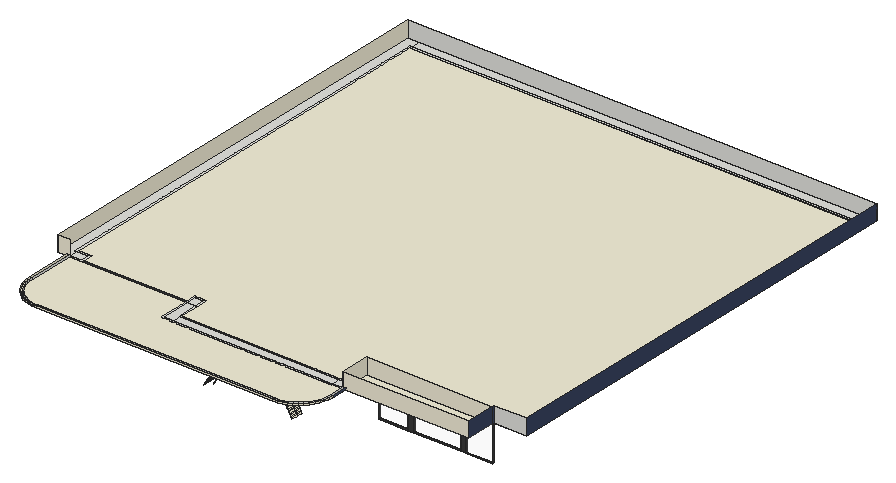
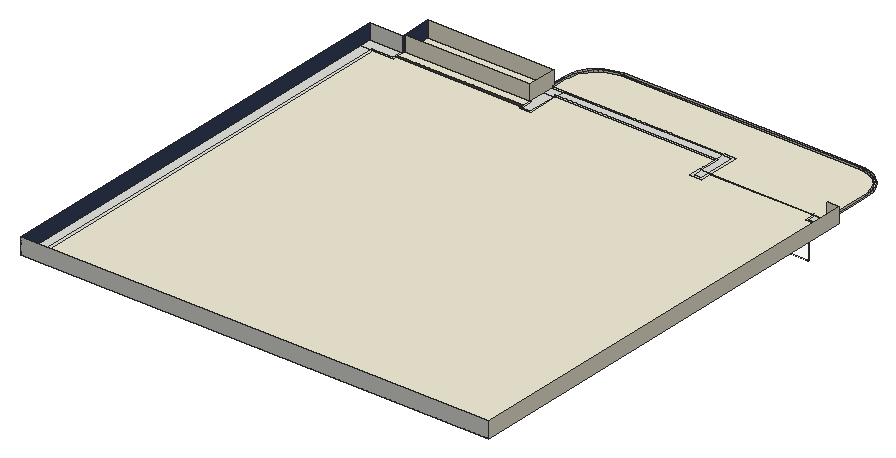
# SketchUp Ruby script. Lengths in inches.
U = 1.inch
M = Sketchup.active_model
def pt(a) = Geom::Point3d.new(a.map { |v| v * U })
def face(e, loops, mat)
  f = e.add_face(loops[0].map { |a| pt(a) })
  loops[1..].each { |l| e.add_face(l.map { |a| pt(a) }).erase! }
  f.material = f.back_material = mat if mat
  f
end
# faces: each face lists its corners as indices into pts; further lists are holes
def faces(e, pts, list, mat = nil) = list.each { |f| face(e, (f[0].is_a?(Array) ? f : [f]).map { |l| l.map { |i| pts[i] } }, mat) }
# xy, xz, yz: faces in a plane at the given z, y or x. An outline is a flat list of corners, or four numbers for a rectangle; further outlines are holes
def ring(l) = l.size == 4 ? [[l[0], l[1]], [l[2], l[1]], [l[2], l[3]], [l[0], l[3]]] : l.each_slice(2).to_a
def flat(e, list, mat, &to3) = list.each { |f| face(e, (f[0].is_a?(Array) ? f : [f]).map { |l| ring(l).map { |u, v| to3.(u, v) } }, mat) }
def xy(e, z, list, mat = nil) = flat(e, list, mat) { |x, y| [x, y, z] }
def xz(e, y, list, mat = nil) = flat(e, list, mat) { |x, z| [x, y, z] }
def yz(e, x, list, mat = nil) = flat(e, list, mat) { |y, z| [x, y, z] }
def lines(e, pts, list) = list.each { |a, b| e.add_line(pt(pts[a]), pt(pts[b])) }
# prism: a flat outline (further loops are holes) pulled along v
def prism(e, loops, v, mat = nil)
  f = face(e, loops, mat); d = Geom::Vector3d.new(v.map { |x| x * U })
  f.pushpull(f.normal.samedirection?(d) ? d.length : -d.length)
end
def box(e, o, s, mat = nil) = prism(e, [[o, [o[0] + s[0], o[1], o[2]], [o[0] + s[0], o[1] + s[1], o[2]], [o[0], o[1] + s[1], o[2]]]], [0, 0, s[2]], mat)
def at(x, y, z, deg = 0) = Geom::Transformation.translation(pt([x, y, z])) * Geom::Transformation.rotation(ORIGIN, Z_AXIS, deg.degrees)
def axes(o, x, y, z) = Geom::Transformation.new([*x, 0, *y, 0, *z, 0, *pt(o).to_a, 1])
def part(name) = M.definitions.add(name)
# library, detail: a bought-in or finely detailed component or shape, given as its bounding box
def library(name, o, s) = part(name).tap { |d| box(d.entities, o, s) }
def detail(e, o, s) = box(e.add_group.entities, o, s)
def put(e, d, t, mat = nil) = e.add_instance(d, t).tap { |i| i.material = mat if mat }
def group(e, t, mat = nil) = e.add_group.tap { |g| g.transformation = t; g.material = mat if mat }.entities
root = M.entities
M.materials.add("0344 AP 9635 Ganges Midnight-N").color = [69, 80, 105]
M.materials.add("0360 AP 9644 Monsoon Midnight-N").color = [56, 67, 95]
M.materials.add("0905 AP 7844 MILD YELLOW").color = [242, 237, 215]
M.materials.add("Glass Clear 001").color = [246, 246, 246]
M.materials["Glass Clear 001"].alpha = 0.1
M.materials.add("[Color M07]").color = [58, 58, 58]
xy(root,86.69,[[46.79,89.9375,64.29,90.25],[67.49,89.9375,95.54,90.25],[98.74,89.9375,118.39,90.25]],"[Color M07]")
xy(root,88.49,[[266.94,94.4375,289.69,95.5],[293.7,94.4375,329.88,95.5],[334.04,94.4375,354.52,95.5]],"[Color M07]")
xy(root,115.63,[[266.94,94.4375,289.69,95.5],[293.7,94.4375,329.88,95.5],[334.04,94.4375,354.52,95.5]])
xy(root,116.26,[[46.79,89.9375,64.29,90.25],[67.49,89.9375,95.54,90.25],[98.74,89.9375,118.39,90.25]])
xy(root,120,[[122.125,65.9375,131.125,65.9375,131.125,67.61,123.8,67.61,123.8,89.9375,122.125,89.9375],[131.125,65.9375,253.5625,67.61],[253.5625,65.9375,262.5625,67.61],[123.8,67.61,131.125,67.61,131.125,73.27,129.45,73.27,129.45,89.9375,123.8,89.9375],[131.125,67.61,253.5625,73.27],
  [253.5625,67.61,262.5625,67.61,262.5625,74.9375,255.23,74.9375,255.23,73.27,253.5625,73.27],[129.45,73.27,131.125,89.9375],[131.125,73.27,253.5625,74.9375],[253.5625,73.27,255.23,74.9375],[253.5625,74.9375,255.23,74.9375,255.23,97.27,260.89,97.27,260.89,88.27,262.5625,88.27,262.5625,98.9375,253.5625,98.9375],
  [255.23,74.9375,262.5625,74.9375,262.5625,88.27,260.89,88.27,260.89,97.27,255.23,97.27],[358.89,88.27,360.57,89.9375],[24,89.9375,31.33,89.9375,31.33,91.61,33,91.61,33,97.27,31.33,97.27,31.33,418.61,33,418.61,33,425.9375,24,425.9375],[31.33,89.9375,33,91.61],[33,89.9375,33,91.61,41.38,91.61,41.38,97.27,33,97.27,33,98.9375,43.05,98.9375,43.05,89.9375],
  [122.125,89.9375,122.125,98.9375,131.125,98.9375,131.125,89.9375,129.45,89.9375,129.45,97.27,123.8,97.27,123.8,89.9375],[123.8,89.9375,129.45,97.27],[358.89,89.9375,358.89,98.9375,376.67,98.9375,376.67,97.27,360.57,97.27,360.57,89.9375],[360.57,89.9375,360.57,97.27,376.67,97.27,376.67,98.9375,384,98.9375,384,89.9375],[33,91.61,41.38,97.27],
  [31.33,97.27,33,418.61],[375,98.9375,376.67,416.9375],[376.67,98.9375,384,416.9375],[33,416.9375,376.67,418.61],[376.67,416.9375,376.67,418.61,33,418.61,33,425.9375,384,425.9375,384,416.9375]])
xy(root,120,[[57,28.27,53.65,28.49,50.36,29.14,47.18,30.22,44.16,31.71,41.37,33.57,38.85,35.79,36.63,38.31,34.77,41.1,33.28,44.11,32.2,47.29,31.55,50.59,31.33,53.9375,31.33,89.9375,33,89.9375,33,53.9375,33.21,50.8,33.82,47.73,34.83,44.75,36.22,41.9375,37.96,39.33,40.03,36.97,42.39,34.9,45,33.15,47.82,31.76,50.79,30.76,53.87,30.14,57,29.9375,238.5625,29.9375,241.7,30.14,244.77,30.76,247.75,31.76,250.5625,33.15,253.17,34.9,255.53,36.97,257.6,39.33,259.35,41.9375,260.74,44.75,261.74,47.73,262.36,50.8,262.5625,53.9375,262.5625,65.9375,264.23,65.9375,264.23,53.9375,264.01,50.59,263.36,47.29,262.28,44.11,260.79,41.1,258.93,38.31,256.71,35.79,254.19,33.57,251.4,31.71,248.39,30.22,245.21,29.14,241.91,28.49,238.5625,28.27],[57,29.9375,53.87,30.14,50.79,30.76,47.82,31.76,45,33.15,42.39,34.9,40.03,36.97,37.96,39.33,36.22,41.9375,34.83,44.75,33.82,47.73,33.21,50.8,33,53.9375,33,89.9375,122.125,89.9375,122.125,65.9375,262.5625,65.9375,262.5625,53.9375,262.36,50.8,261.74,47.73,260.74,44.75,259.35,41.9375,257.6,39.33,255.53,36.97,253.17,34.9,250.5625,33.15,247.75,31.76,244.77,30.76,241.7,30.14,238.5625,29.9375],[262.5625,65.9375,264.23,67.61],[264.23,65.9375,264.23,67.61,262.5625,67.61,262.5625,88.27,358.89,88.27,358.89,65.9375],[131.125,74.9375,131.125,98.9375,122.125,98.9375,122.125,91.4375,43.05,91.4375,43.05,98.9375,33,98.9375,33,416.9375,375,416.9375,375,98.9375,358.89,98.9375,358.89,96.5625,262.5625,96.5625,262.5625,98.9375,253.5625,98.9375,253.5625,74.9375],
  [262.5625,88.27,358.89,94.4375]],"0905 AP 7844 MILD YELLOW")
xy(root,120,[[43.05,89.9375,122.125,91.4375],[262.5625,94.4375,358.89,96.5625]],"[Color M07]")
xz(root,28.27,[[57,120,238.5625,121.25]],"0905 AP 7844 MILD YELLOW")
xz(root,29.9375,[[57,120,238.5625,121.25]])
xz(root,65.9375,[[262.5625,120,358.89,132]],"0905 AP 7844 MILD YELLOW")
xz(root,67.61,[[262.5625,120,264.23,121.25]])
xz(root,88.27,[[262.5625,120,358.89,132]],"0905 AP 7844 MILD YELLOW")
xz(root,89.9375,[[31.33,120,33,121.25],[358.89,120,384,132]])
xz(root,89.9375,[[24,120,31.33,120,31.33,121.25,33,121.25,33,131.3125,32.51,131.3125,32.51,132,24,132]],"0905 AP 7844 MILD YELLOW")
xz(root,89.9375,[[64.29,86.69,67.49,116.26],[95.54,86.69,98.74,116.26]],"[Color M07]")
xz(root,90.25,[[46.79,86.69,64.29,116.26],[67.49,86.69,95.54,116.26],[98.74,86.69,118.39,116.26]],"Glass Clear 001")
xz(root,94.4375,[[289.69,88.49,293.7,115.63],[329.88,88.49,334.04,115.63]],"[Color M07]")
xz(root,95.5,[[266.94,88.49,289.69,115.63],[293.7,88.49,329.88,115.63],[334.04,88.49,354.52,115.63]],"Glass Clear 001")
xz(root,425.9375,[[24,120,384,132]])
yz(root,24,[[89.9375,120,425.9375,132]],"0905 AP 7844 MILD YELLOW")
yz(root,31.33,[[53.9375,120,89.9375,121.25]],"0905 AP 7844 MILD YELLOW")
yz(root,33,[[53.9375,120,89.9375,121.25]])
yz(root,46.79,[[89.9375,86.69,90.25,116.26]],"[Color M07]")
yz(root,64.29,[[89.9375,86.69,90.25,116.26]],"[Color M07]")
yz(root,67.49,[[89.9375,86.69,90.25,116.26]],"[Color M07]")
yz(root,95.54,[[89.9375,86.69,90.25,116.26]],"[Color M07]")
yz(root,98.74,[[89.9375,86.69,90.25,116.26]],"[Color M07]")
yz(root,118.39,[[89.9375,86.69,90.25,116.26]],"[Color M07]")
yz(root,262.5625,[[53.9375,120,65.9375,121.25],[65.9375,120,67.61,121.25]])
yz(root,262.5625,[[67.61,120,88.27,120,88.27,132,65.9375,132,65.9375,121.25,67.61,121.25]],"0905 AP 7844 MILD YELLOW")
yz(root,264.23,[[53.9375,120,67.61,121.25]],"0344 AP 9635 Ganges Midnight-N")
yz(root,266.94,[[94.4375,88.49,95.5,115.63]],"[Color M07]")
yz(root,289.69,[[94.4375,88.49,95.5,115.63]],"[Color M07]")
yz(root,293.7,[[94.4375,88.49,95.5,115.63]],"[Color M07]")
yz(root,329.88,[[94.4375,88.49,95.5,115.63]],"[Color M07]")
yz(root,334.04,[[94.4375,88.49,95.5,115.63]],"[Color M07]")
yz(root,354.52,[[94.4375,88.49,95.5,115.63]],"[Color M07]")
yz(root,358.89,[[65.9375,120,88.27,132],[88.27,120,89.9375,132]],"0360 AP 9644 Monsoon Midnight-N")
yz(root,384,[[89.9375,120,425.9375,132]],"0360 AP 9644 Monsoon Midnight-N")
p = [[159.375,70.75,85.28],[159.71,70.75,85.91],[159.71,70.4375,85.91],[159.375,70.4375,85.28],[155.68,65.9375,85.48],[155.68,70.4375,85.48],
  [156.02,70.4375,86.18],[156.02,65.9375,86.18],[223,65.9375,86.32],[223,70.4375,86.32],[223.42,70.4375,85.48],[223.42,65.9375,85.48],
  [156.02,70.75,86.18],[155.68,70.75,85.48],[219.17,70.75,86.28],[219.59,70.75,85.54],[219.59,70.4375,85.54],[219.17,70.4375,86.28],
  [223.42,70.75,85.48],[223,70.75,86.32],[156.02,74.9375,86.18],[155.68,74.9375,85.48],[223.42,74.9375,85.48],[223,74.9375,86.32],
  [160.07,70.75,86.53],[160.07,70.4375,86.53],[156.38,70.4375,86.87],[156.38,65.9375,86.87],[156.38,70.75,86.87],[156.38,74.9375,86.87],
  [222.57,65.9375,87.15],[222.57,70.4375,87.15],[218.74,70.75,87.02],[218.74,70.4375,87.02],[222.57,70.75,87.15],[222.57,74.9375,87.15],
  [160.43,70.75,87.14],[160.43,70.4375,87.14],[156.76,70.4375,87.56],[156.76,65.9375,87.56],[156.76,70.75,87.56],[156.76,74.9375,87.56],
  [218.29,70.75,87.74],[218.29,70.4375,87.74],[222.11,65.9375,87.97],[222.11,70.4375,87.97],[160.8125,70.75,87.74],[160.8125,70.4375,87.74],
  [222.11,70.75,87.97],[222.11,74.9375,87.97],[157.15,70.4375,88.24],[157.15,65.9375,88.24],[157.15,70.75,88.24],[157.15,74.9375,88.24],
  [161.2,70.75,88.33],[161.2,70.4375,88.33],[217.82,70.75,88.45],[217.82,70.4375,88.45],[221.63,65.9375,88.77],[221.63,70.4375,88.77],
  [221.63,70.75,88.77],[221.63,74.9375,88.77],[157.55,70.4375,88.91],[157.55,65.9375,88.91],[157.55,70.75,88.91],[157.55,74.9375,88.91],
  [161.6,70.75,88.92],[161.6,70.4375,88.92],[217.33,70.75,89.15],[217.33,70.4375,89.15],[221.13,65.9375,89.57],[221.13,70.4375,89.57],
  [221.13,70.75,89.57],[221.13,74.9375,89.57],[157.96,70.4375,89.57],[157.96,65.9375,89.57],[157.96,70.75,89.57],[162.02,70.75,89.5],
  [162.02,70.4375,89.5],[157.96,74.9375,89.57],[216.82,70.75,89.84],[216.82,70.4375,89.84],[162.45,70.75,90.07],[162.45,70.4375,90.07],
  [158.39,70.4375,90.22],[158.39,65.9375,90.22],[220.62,65.9375,90.35],[220.62,70.4375,90.35],[158.39,70.75,90.22],[220.62,70.75,90.35],
  [158.39,74.9375,90.22],[220.62,74.9375,90.35],[216.3,70.75,90.51],[216.3,70.4375,90.51],[162.89,70.75,90.625],[162.89,70.4375,90.625],
  [158.84,70.4375,90.87],[158.84,65.9375,90.87],[158.84,70.75,90.87],[158.84,74.9375,90.87],[220.08,65.9375,91.12],[220.08,70.4375,91.12],
  [220.08,70.75,91.12],[220.08,74.9375,91.12],[215.76,70.75,91.18],[215.76,70.4375,91.18],[163.34,70.75,91.18],[163.34,70.4375,91.18],
  [159.29,70.4375,91.5],[159.29,65.9375,91.5],[159.29,70.75,91.5],[159.29,74.9375,91.5],[219.52,65.9375,91.88],[219.52,70.4375,91.88],
  [219.52,70.75,91.88],[219.52,74.9375,91.88],[163.8,70.75,91.72],[163.8,70.4375,91.72],[215.2,70.75,91.82],[215.2,70.4375,91.82],
  [159.76,70.4375,92.125],[159.76,65.9375,92.125],[159.76,70.75,92.125],[159.76,74.9375,92.125],[164.27,70.75,92.25],[164.27,70.4375,92.25],
  [214.63,70.75,92.46],[214.63,70.4375,92.46],[218.95,65.9375,92.62],[218.95,70.4375,92.62],[218.95,70.75,92.62],[218.95,74.9375,92.62],
  [160.25,70.4375,92.74],[160.25,65.9375,92.74],[160.25,70.75,92.74],[160.25,74.9375,92.74],[164.76,70.75,92.77],[164.76,70.4375,92.77],
  [214.05,70.75,93.08],[214.05,70.4375,93.08],[218.36,65.9375,93.35],[218.36,70.4375,93.35],[218.36,70.75,93.35],[218.36,74.9375,93.35],
  [160.74,70.4375,93.35],[160.74,65.9375,93.35],[160.74,70.75,93.35],[160.74,74.9375,93.35],[165.25,70.75,93.28],[165.25,70.4375,93.28],
  [213.44,70.75,93.68],[213.44,70.4375,93.68],[161.25,70.4375,93.94],[161.25,65.9375,93.94],[217.75,65.9375,94.06],[217.75,70.4375,94.06],
  [161.25,70.75,93.94],[165.76,70.75,93.78],[165.76,70.4375,93.78],[217.75,70.75,94.06],[161.25,74.9375,93.94],[217.75,74.9375,94.06],
  [212.83,70.75,94.27],[212.83,70.4375,94.27],[166.27,70.75,94.27],[166.27,70.4375,94.27],[161.77,70.4375,94.53],[161.77,65.9375,94.53],
  [161.77,70.75,94.53],[161.77,74.9375,94.53],[217.12,65.9375,94.76],[217.12,70.4375,94.76],[217.12,70.75,94.76],[217.12,74.9375,94.76],
  [166.8,70.75,94.75],[166.8,70.4375,94.75],[212.19,70.75,94.85],[212.19,70.4375,94.85],[162.3,70.4375,95.1],[162.3,65.9375,95.1],
  [162.3,70.75,95.1],[162.3,74.9375,95.1],[216.47,65.9375,95.4375],[216.47,70.4375,95.4375],[167.33,70.75,95.22],[167.33,70.4375,95.22],
  [211.55,70.75,95.4],[211.55,70.4375,95.4],[216.47,70.75,95.4375],[216.47,74.9375,95.4375],[162.84,70.4375,95.66],[162.84,65.9375,95.66],
  [162.84,70.75,95.66],[162.84,74.9375,95.66],[167.88,70.75,95.68],[167.88,70.4375,95.68],[215.81,65.9375,96.1],[215.81,70.4375,96.1],
  [210.89,70.75,95.94],[210.89,70.4375,95.94],[215.81,70.75,96.1],[215.81,74.9375,96.1],[163.4,70.4375,96.21],[163.4,65.9375,96.21],
  [163.4,70.75,96.21],[168.43,70.75,96.12],[168.43,70.4375,96.12],[163.4,74.9375,96.21],[210.21,70.75,96.47],[210.21,70.4375,96.47],
  [215.13,65.9375,96.75],[215.13,70.4375,96.75],[169,70.75,96.55],[169,70.4375,96.55],[215.13,70.75,96.75],[215.13,74.9375,96.75],
  [163.97,70.4375,96.75],[163.97,65.9375,96.75],[163.97,70.75,96.75],[163.97,74.9375,96.75],[209.53,70.75,96.98],[209.53,70.4375,96.98],
  [169.57,70.75,96.98],[169.57,70.4375,96.98],[164.54,70.4375,97.28],[164.54,65.9375,97.28],[214.4375,65.9375,97.38],[214.4375,70.4375,97.38],
  [164.54,70.75,97.28],[214.4375,70.75,97.38],[164.54,74.9375,97.28],[214.4375,74.9375,97.38],[170.15,70.75,97.39],[170.15,70.4375,97.39],
  [208.83,70.75,97.47],[208.83,70.4375,97.47],[165.13,70.4375,97.79],[165.13,65.9375,97.79],[165.13,70.75,97.79],[165.13,74.9375,97.79],
  [213.73,65.9375,97.99],[213.73,70.4375,97.99],[170.74,70.75,97.78],[170.74,70.4375,97.78],[213.73,70.75,97.99],[213.73,74.9375,97.99],
  [208.12,70.75,97.94],[208.12,70.4375,97.94],[165.73,70.4375,98.29],[165.73,65.9375,98.29],[165.73,70.75,98.29],[171.34,70.75,98.17],
  [171.34,70.4375,98.17],[165.73,74.9375,98.29],[207.4,70.75,98.4],[207.4,70.4375,98.4],[213,65.9375,98.59],[213,70.4375,98.59],
  [213,70.75,98.59],[213,74.9375,98.59],[171.94,70.75,98.54],[171.94,70.4375,98.54],[166.34,70.4375,98.78],[166.34,65.9375,98.78],
  [166.34,70.75,98.78],[166.34,74.9375,98.78],[206.66,70.75,98.83],[206.66,70.4375,98.83],[172.56,70.75,98.9],[172.56,70.4375,98.9],
  [212.26,65.9375,99.16],[212.26,70.4375,99.16],[212.26,70.75,99.16],[212.26,74.9375,99.16],[166.96,70.4375,99.26],[166.96,65.9375,99.26],
  [166.96,70.75,99.26],[205.92,70.75,99.25],[205.92,70.4375,99.25],[166.96,74.9375,99.26],[173.18,70.75,99.25],[173.18,70.4375,99.25],
  [211.51,65.9375,99.72],[211.51,70.4375,99.72],[211.51,70.75,99.72],[211.51,74.9375,99.72],[167.59,70.4375,99.72],[167.59,65.9375,99.72],
  [167.59,70.75,99.72],[173.81,70.75,99.58],[173.81,70.4375,99.58],[205.16,70.75,99.65],[205.16,70.4375,99.65],[167.59,74.9375,99.72],
  [174.44,70.75,99.91],[174.44,70.4375,99.91],[204.4,70.75,100.03],[204.4,70.4375,100.03],[168.23,70.4375,100.17],[168.23,65.9375,100.17],
  [210.74,65.9375,100.26],[210.74,70.4375,100.26],[168.23,70.75,100.17],[210.74,70.75,100.26],[168.23,74.9375,100.17],[210.74,74.9375,100.26],
  [175.08,70.75,100.21],[175.08,70.4375,100.21],[203.63,70.75,100.39],[203.63,70.4375,100.39],[168.875,70.4375,100.61],[168.875,65.9375,100.61],
  [168.875,70.75,100.61],[175.73,70.75,100.51],[175.73,70.4375,100.51],[168.875,74.9375,100.61],[209.96,65.9375,100.78],[209.96,70.4375,100.78],
  [209.96,70.75,100.78],[209.96,74.9375,100.78],[202.85,70.75,100.73],[202.85,70.4375,100.73],[176.38,70.75,100.79],[176.38,70.4375,100.79],
  [169.53,70.4375,101.03],[169.53,65.9375,101.03],[169.53,70.75,101.03],[169.53,74.9375,101.03],[202.06,70.75,101.06],[202.06,70.4375,101.06],
  [209.16,65.9375,101.28],[209.16,70.4375,101.28],[177.04,70.75,101.06],[177.04,70.4375,101.06],[209.16,70.75,101.28],[209.16,74.9375,101.28],
  [170.2,70.4375,101.44],[170.2,65.9375,101.44],[170.2,70.75,101.44],[170.2,74.9375,101.44],[177.71,70.75,101.31],[177.71,70.4375,101.31],
  [201.26,70.75,101.36],[201.26,70.4375,101.36],[208.36,65.9375,101.76],[208.36,70.4375,101.76],[178.375,70.75,101.55],[178.375,70.4375,101.55],
  [208.36,70.75,101.76],[208.36,74.9375,101.76],[170.875,70.4375,101.84],[170.875,65.9375,101.84],[170.875,70.75,101.84],[200.45,70.75,101.64],
  [200.45,70.4375,101.64],[170.875,74.9375,101.84],[179.05,70.75,101.78],[179.05,70.4375,101.78],[199.64,70.75,101.9],[199.64,70.4375,101.9],
  [171.56,70.4375,102.22],[171.56,65.9375,102.22],[207.54,65.9375,102.22],[207.54,70.4375,102.22],[171.56,70.75,102.22],[179.73,70.75,101.99],
  [179.73,70.4375,101.99],[207.54,70.75,102.22],[171.56,74.9375,102.22],[207.54,74.9375,102.22],[198.82,70.75,102.15],[198.82,70.4375,102.15],
  [180.41,70.75,102.18],[180.41,70.4375,102.18],[198,70.75,102.37],[198,70.4375,102.37],[172.25,70.4375,102.59],[172.25,65.9375,102.59],
  [206.71,65.9375,102.66],[206.71,70.4375,102.66],[172.25,70.75,102.59],[181.1,70.75,102.37],[181.1,70.4375,102.37],[206.71,70.75,102.66],
  [172.25,74.9375,102.59],[206.71,74.9375,102.66],[181.79,70.75,102.54],[181.79,70.4375,102.54],[197.17,70.75,102.57],[197.17,70.4375,102.57],
  [182.49,70.75,102.69],[182.49,70.4375,102.69],[172.94,70.4375,102.94],[172.94,65.9375,102.94],[172.94,70.75,102.94],[196.33,70.75,102.75],
  [196.33,70.4375,102.75],[172.94,74.9375,102.94],[205.87,65.9375,103.08],[205.87,70.4375,103.08],[183.18,70.75,102.83],[183.18,70.4375,102.83],
  [195.49,70.75,102.91],[195.49,70.4375,102.91],[205.87,70.75,103.08],[205.87,74.9375,103.08],[183.88,70.75,102.96],[183.88,70.4375,102.96],
  [173.65,70.4375,103.28],[173.65,65.9375,103.28],[173.65,70.75,103.28],[194.65,70.75,103.04],[194.65,70.4375,103.04],[173.65,74.9375,103.28],
  [184.59,70.75,103.07],[184.59,70.4375,103.07],[193.81,70.75,103.16],[193.81,70.4375,103.16],[205.02,65.9375,103.48],[205.02,70.4375,103.48],
  [185.29,70.75,103.16],[185.29,70.4375,103.16],[205.02,70.75,103.48],[205.02,74.9375,103.48],[186,70.75,103.24],[186,70.4375,103.24],
  [186.71,70.75,103.31],[186.71,70.4375,103.31],[192.96,70.75,103.26],[192.96,70.4375,103.26],[174.36,70.4375,103.6],[174.36,65.9375,103.6],
  [174.36,70.75,103.6],[187.42,70.75,103.36],[187.42,70.4375,103.36],[191.26,70.75,103.39],[192.11,70.75,103.33],[192.11,70.4375,103.33],
  [191.26,70.4375,103.39],[174.36,74.9375,103.6],[188.125,70.75,103.4],[188.125,70.4375,103.4],[188.84,70.75,103.42],[188.84,70.4375,103.42],
  [189.54,70.75,103.43],[189.54,70.4375,103.43],[190.4,70.75,103.42],[190.4,70.4375,103.42],[204.16,65.9375,103.85],[204.16,70.4375,103.85],
  [204.16,70.75,103.85],[204.16,74.9375,103.85],[175.08,70.4375,103.91],[175.08,65.9375,103.91],[175.08,70.75,103.91],[175.08,74.9375,103.91],
  [175.8,70.4375,104.21],[175.8,65.9375,104.21],[203.29,65.9375,104.21],[203.29,70.4375,104.21],[175.8,70.75,104.21],[203.29,70.75,104.21],
  [175.8,74.9375,104.21],[203.29,74.9375,104.21],[176.53,70.4375,104.48],[176.53,65.9375,104.48],[202.42,65.9375,104.54],[202.42,70.4375,104.54],
  [176.53,70.75,104.48],[202.42,70.75,104.54],[176.53,74.9375,104.48],[202.42,74.9375,104.54],[177.27,70.4375,104.75],[177.27,65.9375,104.75],
  [201.53,65.9375,104.85],[201.53,70.4375,104.85],[177.27,70.75,104.75],[201.53,70.75,104.85],[177.27,74.9375,104.75],[201.53,74.9375,104.85],
  [178.01,70.4375,105],[178.01,65.9375,105],[178.01,70.75,105],[178.01,74.9375,105],[200.64,65.9375,105.14],[200.64,70.4375,105.14],
  [200.64,70.75,105.14],[200.64,74.9375,105.14],[178.76,70.4375,105.23],[178.76,65.9375,105.23],[178.76,70.75,105.23],[178.76,74.9375,105.23],
  [199.74,65.9375,105.4],[199.74,70.4375,105.4],[199.74,70.75,105.4],[199.74,74.9375,105.4],[179.51,70.4375,105.45],[179.51,65.9375,105.45],
  [179.51,70.75,105.45],[179.51,74.9375,105.45],[180.26,70.4375,105.65],[180.26,65.9375,105.65],[198.83,65.9375,105.65],[198.83,70.4375,105.65],
  [180.26,70.75,105.65],[198.83,70.75,105.65],[180.26,74.9375,105.65],[198.83,74.9375,105.65],[181.02,70.4375,105.83],[181.02,65.9375,105.83],
  [197.92,65.9375,105.87],[197.92,70.4375,105.87],[181.02,70.75,105.83],[197.92,70.75,105.87],[181.02,74.9375,105.83],[197.92,74.9375,105.87],
  [181.79,70.4375,106],[181.79,65.9375,106],[181.79,70.75,106],[181.79,74.9375,106],[197,65.9375,106.06],[197,70.4375,106.06],
  [197,70.75,106.06],[197,74.9375,106.06],[182.55,70.4375,106.16],[182.55,65.9375,106.16],[182.55,70.75,106.16],[182.55,74.9375,106.16],
  [196.08,65.9375,106.24],[196.08,70.4375,106.24],[196.08,70.75,106.24],[196.08,74.9375,106.24],[183.32,70.4375,106.29],[183.32,65.9375,106.29],
  [195.16,65.9375,106.39],[195.16,70.4375,106.39],[183.32,70.75,106.29],[195.16,70.75,106.39],[183.32,74.9375,106.29],[195.16,74.9375,106.39],
  [184.1,70.4375,106.41],[184.1,65.9375,106.41],[184.1,70.75,106.41],[184.1,74.9375,106.41],[184.87,70.4375,106.52],[184.87,65.9375,106.52],
  [194.23,65.9375,106.52],[194.23,70.4375,106.52],[184.87,70.75,106.52],[194.23,70.75,106.52],[184.87,74.9375,106.52],[194.23,74.9375,106.52],
  [185.65,70.4375,106.61],[185.65,65.9375,106.61],[193.29,65.9375,106.625],[193.29,70.4375,106.625],[185.65,70.75,106.61],[193.29,70.75,106.625],
  [185.65,74.9375,106.61],[193.29,74.9375,106.625],[186.42,70.4375,106.68],[186.42,65.9375,106.68],[192.36,65.9375,106.71],[192.36,70.4375,106.71],
  [186.42,70.75,106.68],[192.36,70.75,106.71],[186.42,74.9375,106.68],[192.36,74.9375,106.71],[187.2,70.4375,106.74],[187.2,65.9375,106.74],
  [187.99,70.4375,106.78],[187.99,65.9375,106.78],[191.42,65.9375,106.77],[191.42,70.4375,106.77],[187.2,70.75,106.74],[187.99,70.75,106.78],
  [191.42,70.75,106.77],[187.2,74.9375,106.74],[187.99,74.9375,106.78],[191.42,74.9375,106.77],[188.77,70.4375,106.8],[188.77,65.9375,106.8],
  [189.55,70.4375,106.8125],[189.55,65.9375,106.8125],[190.49,70.4375,106.8],[190.49,65.9375,106.8],[188.77,70.75,106.8],[189.55,70.75,106.8125],
  [190.49,70.75,106.8],[188.77,74.9375,106.8],[189.55,74.9375,106.8125],[190.49,74.9375,106.8],[53.65,28.49,120],[57,28.27,120],
  [57,28.27,121.25],[53.65,28.49,121.25],[238.5625,28.27,120],[241.91,28.49,120],[241.91,28.49,121.25],[238.5625,28.27,121.25],
  [50.36,29.14,120],[50.36,29.14,121.25],[245.21,29.14,120],[245.21,29.14,121.25],[47.18,30.22,120],[47.18,30.22,121.25],
  [248.39,30.22,120],[248.39,30.22,121.25],[53.87,30.14,120],[57,29.9375,120],[57,29.9375,121.25],[53.87,30.14,121.25],
  [238.5625,29.9375,120],[241.7,30.14,120],[241.7,30.14,121.25],[238.5625,29.9375,121.25],[50.79,30.76,120],[50.79,30.76,121.25],
  [244.77,30.76,120],[244.77,30.76,121.25],[44.16,31.71,120],[44.16,31.71,121.25],[251.4,31.71,120],[251.4,31.71,121.25],
  [47.82,31.76,120],[47.82,31.76,121.25],[247.75,31.76,120],[247.75,31.76,121.25],[41.37,33.57,120],[41.37,33.57,121.25],
  [254.19,33.57,120],[254.19,33.57,121.25],[45,33.15,120],[45,33.15,121.25],[250.5625,33.15,120],[250.5625,33.15,121.25],
  [42.39,34.9,120],[42.39,34.9,121.25],[253.17,34.9,120],[253.17,34.9,121.25],[38.85,35.79,120],[38.85,35.79,121.25],
  [256.71,35.79,120],[256.71,35.79,121.25],[40.03,36.97,120],[40.03,36.97,121.25],[255.53,36.97,120],[255.53,36.97,121.25],
  [36.63,38.31,120],[36.63,38.31,121.25],[258.93,38.31,120],[258.93,38.31,121.25],[37.96,39.33,120],[37.96,39.33,121.25],
  [257.6,39.33,120],[257.6,39.33,121.25],[34.77,41.1,120],[34.77,41.1,121.25],[260.79,41.1,120],[260.79,41.1,121.25],
  [36.22,41.9375,120],[36.22,41.9375,121.25],[259.35,41.9375,120],[259.35,41.9375,121.25],[33.28,44.11,120],[33.28,44.11,121.25],
  [262.28,44.11,120],[262.28,44.11,121.25],[34.83,44.75,120],[34.83,44.75,121.25],[260.74,44.75,120],[260.74,44.75,121.25],
  [32.2,47.29,120],[32.2,47.29,121.25],[263.36,47.29,120],[263.36,47.29,121.25],[33.82,47.73,120],[33.82,47.73,121.25],
  [261.74,47.73,120],[261.74,47.73,121.25],[31.55,50.59,120],[31.55,50.59,121.25],[264.01,50.59,120],[264.01,50.59,121.25],
  [33.21,50.8,120],[33.21,50.8,121.25],[262.36,50.8,120],[262.36,50.8,121.25],[31.33,53.9375,120],[31.33,53.9375,121.25],
  [264.23,53.9375,120],[264.23,53.9375,121.25],[33,53.9375,120],[33,53.9375,121.25],[262.5625,53.9375,120],[262.5625,53.9375,121.25]]
faces(root,p,[[0,1,2,3],[12,13,5,6],[14,15,16,17],[18,19,9,10],[1,24,25,2],[28,12,6,26],[32,14,17,33],[19,34,31,9],
  [24,36,37,25],[40,28,26,38],[42,32,33,43],[36,46,47,37],[34,48,45,31],[52,40,38,50],[46,54,55,47],[56,42,43,57],
  [48,60,59,45],[64,52,50,62],[54,66,67,55],[68,56,57,69],[60,72,71,59],[76,64,62,74],[66,77,78,67],[80,68,69,81],
  [77,82,83,78],[88,76,74,84],[72,89,87,71],[92,80,81,93],[82,94,95,83],[98,88,84,96],[89,102,101,87],[104,92,93,105],
  [94,106,107,95],[110,98,96,108],[102,114,113,101],[106,116,117,107],[118,104,105,119],[122,110,108,120],[116,124,125,117],[126,118,119,127],
  [114,130,129,113],[134,122,120,132],[124,136,137,125],[138,126,127,139],[130,142,141,129],[146,134,132,144],[136,148,149,137],[150,138,139,151],
  [156,146,144,152],[148,157,158,149],[142,159,155,141],[162,150,151,163],[157,164,165,158],[168,156,152,166],[159,172,171,155],[164,174,175,165],
  [176,162,163,177],[180,168,166,178],[174,184,185,175],[186,176,177,187],[172,188,183,171],[192,180,178,190],[184,194,195,185],[198,186,187,199],
  [188,200,197,183],[204,192,190,202],[194,205,206,195],[208,198,199,209],[205,212,213,206],[200,214,211,197],[218,204,202,216],[220,208,209,221],
  [212,222,223,213],[228,218,216,224],[214,229,227,211],[222,232,233,223],[234,220,221,235],[238,228,224,236],[232,242,243,233],[229,244,241,227],
  [246,234,235,247],[250,238,236,248],[242,251,252,243],[254,246,247,255],[244,258,257,241],[251,260,261,252],[264,250,248,262],[266,254,255,267],
  [260,268,269,261],[258,272,271,257],[276,264,262,274],[277,266,267,278],[268,280,281,269],[272,284,283,271],[288,276,274,286],[280,289,290,281],
  [291,277,278,292],[289,294,295,290],[296,291,292,297],[302,288,286,298],[284,303,301,283],[294,306,307,295],[308,296,297,309],[312,302,298,310],
  [306,313,314,307],[303,318,317,301],[320,308,309,321],[313,322,323,314],[326,312,310,324],[328,320,321,329],[322,332,333,323],[318,334,331,317],
  [338,326,324,336],[332,340,341,333],[342,328,329,343],[340,346,347,341],[334,348,345,331],[352,338,336,350],[353,342,343,354],[346,356,357,347],
  [358,353,354,359],[364,352,350,360],[356,365,366,357],[348,367,363,345],[370,358,359,371],[365,372,373,366],[374,370,371,375],[380,364,360,376],
  [372,381,382,373],[367,383,379,363],[381,386,387,382],[388,374,375,389],[386,390,391,387],[394,380,376,392],[395,388,389,396],[390,400,401,391],
  [402,395,396,403],[383,404,399,379],[400,406,407,401],[410,394,392,408],[411,402,403,412],[406,414,415,407],[416,411,412,417],[414,420,421,415],
  [404,422,419,399],[420,424,425,421],[424,426,427,425],[428,416,417,429],[432,410,408,430],[426,433,434,427],[435,436,437,438],[436,428,429,437],
  [433,440,441,434],[440,442,443,441],[442,444,445,443],[444,446,447,445],[446,435,438,447],[422,450,449,419],[454,432,430,452],[460,454,452,456],
  [450,461,459,449],[468,460,456,464],[461,469,467,459],[476,468,464,472],[469,477,475,467],[482,476,472,480],[477,486,485,475],[490,482,480,488],
  [486,494,493,485],[498,490,488,496],[504,498,496,500],[494,505,503,493],[512,504,500,508],[505,513,511,503],[518,512,508,516],[513,522,521,511],
  [526,518,516,524],[522,530,529,521],[536,526,524,532],[530,537,535,529],[542,536,532,540],[548,542,540,544],[537,549,547,535],[556,548,544,552],
  [549,557,555,547],[564,556,552,560],[557,565,563,555],[574,564,560,568],[575,574,568,570],[565,576,573,563],[586,575,570,580],[587,586,580,582],
  [588,587,582,584],[576,588,584,573]],"[Color M07]")
faces(root,p,[[4,5,6,7],[8,9,10,11],[20,12,13,21],[22,18,19,23],[7,6,26,27],[29,28,12,20],[30,31,9,8],[23,19,34,35],
  [27,26,38,39],[41,40,28,29],[44,45,31,30],[35,34,48,49],[39,38,50,51],[53,52,40,41],[58,59,45,44],[49,48,60,61],
  [51,50,62,63],[65,64,52,53],[70,71,59,58],[61,60,72,73],[63,62,74,75],[79,76,64,65],[75,74,84,85],[86,87,71,70],
  [90,88,76,79],[73,72,89,91],[85,84,96,97],[99,98,88,90],[100,101,87,86],[91,89,102,103],[97,96,108,109],[111,110,98,99],
  [112,113,101,100],[103,102,114,115],[109,108,120,121],[123,122,110,111],[128,129,113,112],[115,114,130,131],[121,120,132,133],[135,134,122,123],
  [140,141,129,128],[131,130,142,143],[133,132,144,145],[147,146,134,135],[145,144,152,153],[154,155,141,140],[160,156,146,147],[143,142,159,161],
  [153,152,166,167],[169,168,156,160],[170,171,155,154],[161,159,172,173],[167,166,178,179],[181,180,168,169],[182,183,171,170],[173,172,188,189],
  [179,178,190,191],[193,192,180,181],[196,197,183,182],[189,188,200,201],[191,190,202,203],[207,204,192,193],[210,211,197,196],[201,200,214,215],
  [203,202,216,217],[219,218,204,207],[217,216,224,225],[226,227,211,210],[230,228,218,219],[215,214,229,231],[225,224,236,237],[239,238,228,230],
  [240,241,227,226],[231,229,244,245],[237,236,248,249],[253,250,238,239],[256,257,241,240],[245,244,258,259],[249,248,262,263],[265,264,250,253],
  [270,271,257,256],[259,258,272,273],[263,262,274,275],[279,276,264,265],[282,283,271,270],[273,272,284,285],[275,274,286,287],[293,288,276,279],
  [287,286,298,299],[300,301,283,282],[304,302,288,293],[285,284,303,305],[299,298,310,311],[315,312,302,304],[316,317,301,300],[305,303,318,319],
  [311,310,324,325],[327,326,312,315],[330,331,317,316],[319,318,334,335],[325,324,336,337],[339,338,326,327],[344,345,331,330],[335,334,348,349],
  [337,336,350,351],[355,352,338,339],[351,350,360,361],[362,363,345,344],[368,364,352,355],[349,348,367,369],[361,360,376,377],[378,379,363,362],
  [384,380,364,368],[369,367,383,385],[377,376,392,393],[397,394,380,384],[398,399,379,378],[385,383,404,405],[393,392,408,409],[413,410,394,397],
  [418,419,399,398],[405,404,422,423],[409,408,430,431],[439,432,410,413],[448,449,419,418],[423,422,450,451],[431,430,452,453],[455,454,432,439],
  [453,452,456,457],[458,459,449,448],[462,460,454,455],[451,450,461,463],[457,456,464,465],[466,467,459,458],[470,468,460,462],[463,461,469,471],
  [465,464,472,473],[474,475,467,466],[478,476,468,470],[471,469,477,479],[473,472,480,481],[483,482,476,478],[484,485,475,474],[479,477,486,487],
  [481,480,488,489],[491,490,482,483],[492,493,485,484],[487,486,494,495],[489,488,496,497],[499,498,490,491],[497,496,500,501],[502,503,493,492],
  [506,504,498,499],[495,494,505,507],[501,500,508,509],[510,511,503,502],[514,512,504,506],[507,505,513,515],[509,508,516,517],[519,518,512,514],
  [520,521,511,510],[515,513,522,523],[517,516,524,525],[527,526,518,519],[528,529,521,520],[523,522,530,531],[525,524,532,533],[534,535,529,528],
  [538,536,526,527],[531,530,537,539],[533,532,540,541],[543,542,536,538],[541,540,544,545],[546,547,535,534],[550,548,542,543],[539,537,549,551],
  [545,544,552,553],[554,555,547,546],[558,556,548,550],[551,549,557,559],[553,552,560,561],[562,563,555,554],[566,564,556,558],[559,557,565,567],
  [561,560,568,569],[569,568,570,571],[572,573,563,562],[577,574,564,566],[578,575,574,577],[567,565,576,579],[571,570,580,581],[581,580,582,583],
  [583,582,584,585],[585,584,573,572],[589,586,575,578],[590,587,586,589],[591,588,587,590],[579,576,588,591],[592,593,594,595],[596,597,598,599],
  [600,592,595,601],[597,602,603,598],[604,600,601,605],[602,606,607,603],[620,604,605,621],[606,622,623,607],[628,620,621,629],[622,630,631,623],
  [640,628,629,641],[630,642,643,631],[648,640,641,649],[642,650,651,643],[656,648,649,657],[650,658,659,651],[664,656,657,665],[658,666,667,659],
  [672,664,665,673],[666,674,675,667],[680,672,673,681],[674,682,683,675],[688,680,681,689],[682,690,691,683]],"0905 AP 7844 MILD YELLOW")
faces(root,p,[[608,609,610,611],[612,613,614,615],[616,608,611,617],[613,618,619,614],[624,616,617,625],[618,626,627,619],[632,624,625,633],[626,634,635,627],
  [636,632,633,637],[634,638,639,635],[644,636,637,645],[638,646,647,639],[652,644,645,653],[646,654,655,647],[660,652,653,661],[654,662,663,655],
  [668,660,661,669],[662,670,671,663],[676,668,669,677],[670,678,679,671],[684,676,677,685],[678,686,687,679],[692,684,685,693],[686,694,695,687]])
